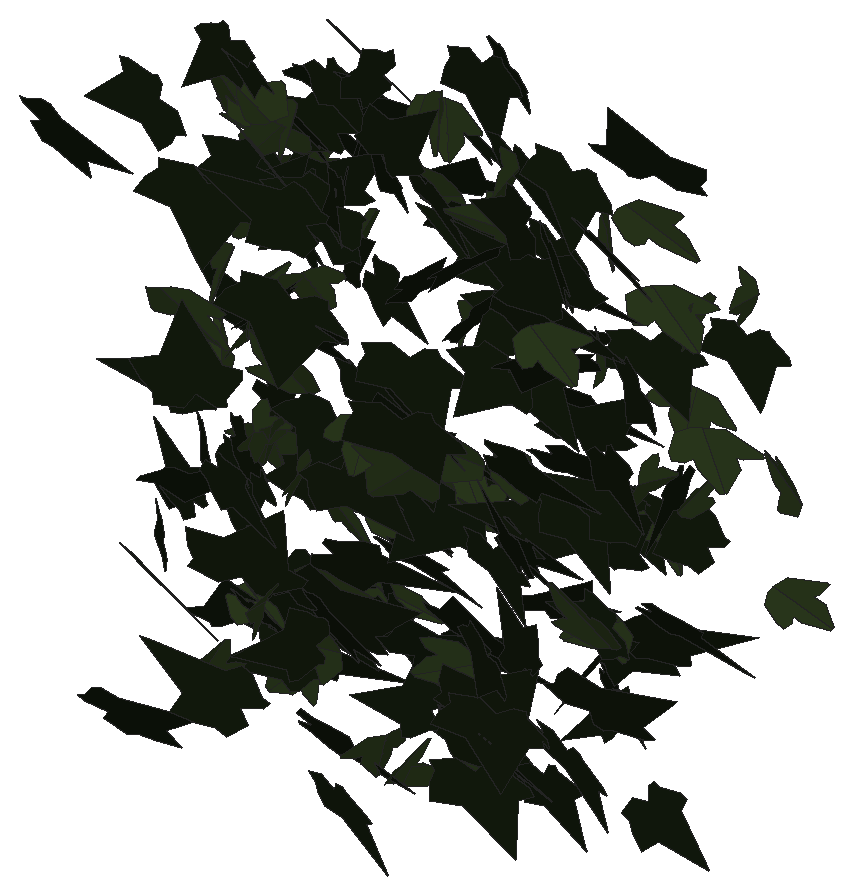
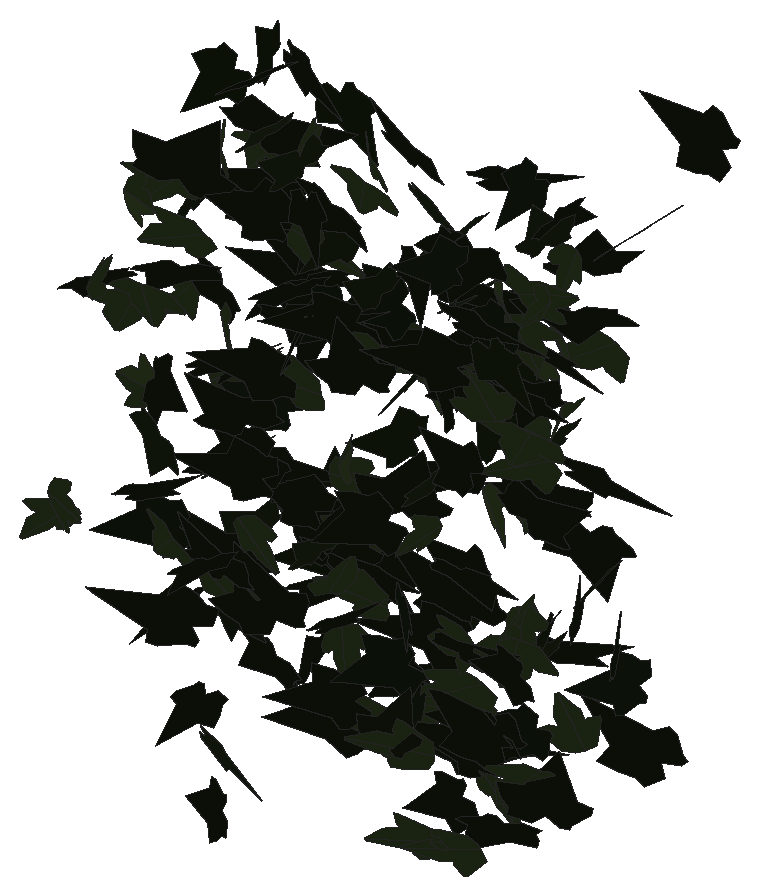
# SketchUp Ruby script. Lengths in millimetres.
U = 1.mm
M = Sketchup.active_model
def pt(a) = Geom::Point3d.new(a.map { |v| v * U })
def face(e, loops, mat)
  f = e.add_face(loops[0].map { |a| pt(a) })
  loops[1..].each { |l| e.add_face(l.map { |a| pt(a) }).erase! }
  f.material = f.back_material = mat if mat
  f
end
# faces: each face lists its corners as indices into pts; further lists are holes
def faces(e, pts, list, mat = nil) = list.each { |f| face(e, (f[0].is_a?(Array) ? f : [f]).map { |l| l.map { |i| pts[i] } }, mat) }
# xy, xz, yz: faces in a plane at the given z, y or x. An outline is a flat list of corners, or four numbers for a rectangle; further outlines are holes
def ring(l) = l.size == 4 ? [[l[0], l[1]], [l[2], l[1]], [l[2], l[3]], [l[0], l[3]]] : l.each_slice(2).to_a
def flat(e, list, mat, &to3) = list.each { |f| face(e, (f[0].is_a?(Array) ? f : [f]).map { |l| ring(l).map { |u, v| to3.(u, v) } }, mat) }
def xy(e, z, list, mat = nil) = flat(e, list, mat) { |x, y| [x, y, z] }
def xz(e, y, list, mat = nil) = flat(e, list, mat) { |x, z| [x, y, z] }
def yz(e, x, list, mat = nil) = flat(e, list, mat) { |y, z| [x, y, z] }
def lines(e, pts, list) = list.each { |a, b| e.add_line(pt(pts[a]), pt(pts[b])) }
# prism: a flat outline (further loops are holes) pulled along v
def prism(e, loops, v, mat = nil)
  f = face(e, loops, mat); d = Geom::Vector3d.new(v.map { |x| x * U })
  f.pushpull(f.normal.samedirection?(d) ? d.length : -d.length)
end
def box(e, o, s, mat = nil) = prism(e, [[o, [o[0] + s[0], o[1], o[2]], [o[0] + s[0], o[1] + s[1], o[2]], [o[0], o[1] + s[1], o[2]]]], [0, 0, s[2]], mat)
def at(x, y, z, deg = 0) = Geom::Transformation.translation(pt([x, y, z])) * Geom::Transformation.rotation(ORIGIN, Z_AXIS, deg.degrees)
def axes(o, x, y, z) = Geom::Transformation.new([*x, 0, *y, 0, *z, 0, *pt(o).to_a, 1])
def part(name) = M.definitions.add(name)
# library, detail: a bought-in or finely detailed component or shape, given as its bounding box
def library(name, o, s) = part(name).tap { |d| box(d.entities, o, s) }
def detail(e, o, s) = box(e.add_group.entities, o, s)
def put(e, d, t, mat = nil) = e.add_instance(d, t).tap { |i| i.material = mat if mat }
def group(e, t, mat = nil) = e.add_group.tap { |g| g.transformation = t; g.material = mat if mat }.entities
root = M.entities
M.materials.add("efeu1").color = [18, 25, 13]
M.materials.add("efeu2").color = [43, 57, 29]
c1 = part("ivyleaf_9")
p = [[39.1,54.8,31.7],[34.5,51.8,30.2],[-5.3,25.2,17.3],[-17.9,28.3,20.9],[-21.6,21.7,17],[-20.2,4.3,5.3],
  [-22.9,-0.3,2.5],[-17.1,-4,-0.6],[-2,-2.1,-1.2],[-0.7,-15.4,-10.1],[16.6,-22.3,-16.7],[21.1,-15.1,-12.5],
  [32.7,-10.7,-11],[46.1,-1.8,-6.6],[30.8,11.2,3.8]]
faces(c1.entities,p,[[0,1,2,3,4,5,6,7,8,9,10,11,12,13,14]],"efeu1")
c2 = part("ivyleaf_10")
p = [[0,12.8,-0.8],[-1.5,51.3,-10.9],[-4.9,51,-11.6],[-13.6,26.5,-7.3],[-13.2,15.9,-4.6],[-21.1,19.3,-7.2],
  [-29.5,16.3,-8.3],[-29.2,8.3,-6.2],[-19.7,-9.8,0.5],[-7.6,-13,4],[1,-12.2,5.8],[-0.4,51.1,-11.1],
  [-1.5,51.1,-10.9],[1,-12.4,5.9],[16.9,-12.4,3.5],[35.1,9.1,-5.1],[35,12.9,-6.1],[20.5,16.4,-4.9],
  [15.8,15,-3.8],[15.3,27.6,-7.1],[12.8,31.3,-7.8]]
faces(c2.entities,p,[[0,1,2,3,4,5,6,7,8,9,10],[11,12,0,13,14,15,16,17,18,19,20]],"efeu2")
put(root,c1,axes([5355,619.4,1867.7],[-0.14381,0.13814,1.11559],[-0.4553,-1.09447,0.11932],[2.0904,-0.22888,0.10273]))
put(root,c1,axes([5360.8,766.3,1691.6],[1.70624,0.24409,0.77946],[-1.42606,-0.21489,0.92911],[0.61874,-1.16838,-0.00805]))
put(root,c1,axes([5329.5,599.9,1839.7],[1.79661,-0.87085,0.22516],[0.30156,-0.16029,-1.28429],[1.68513,0.95714,-0.01022]))
put(root,c1,axes([5332.9,867,1972.2],[0.18817,-0.09167,-1.07306],[2.04965,0.00299,0.09898],[-0.01032,-1.0776,0.09155]))
put(root,c1,axes([5360,701.5,1966.5],[-0.00869,-0.12447,1.15708],[-0.36189,-1.14146,-0.12354],[2.1851,-0.18954,-0.01586]))
put(root,c1,axes([5352.7,875.9,1723.1],[-0.57705,-0.64679,-0.80667],[0.74353,0.70665,-0.71344],[1.82193,-0.49324,0.03566]))
put(root,c1,axes([5378.1,577.2,2538.2],[0.57772,-1.14595,-0.77761],[0.39902,-0.74886,1.18544],[-2.60531,-0.36881,0.00913]))
put(root,c1,axes([5408.1,745.4,2149.6],[0.33354,-0.23641,1.17944],[-1.48326,0.88558,0.29331],[-1.74387,-0.79845,-0.0239]))
put(root,c2,axes([5356,812.5,2329.7],[2.19955,0.23269,0.39445],[0.73662,0.0761,-1.1789],[-0.46594,1.2188,-0.0017]))
put(root,c1,axes([5381.4,737.3,1975.6],[1.09422,-0.48773,-0.98454],[-1.42174,0.64132,-0.75394],[1.53341,0.94265,0.00353]))
put(root,c2,axes([5362.2,782.7,2273.4],[-0.9382,-0.24559,-0.99546],[1.69083,0.44907,-0.55074],[0.97411,-1.01601,-0.0028]))
put(root,c2,axes([5397.6,665.5,2546.6],[-1.50843,0.82441,0.15893],[-0.20941,0.11468,-1.1436],[-1.58412,-0.80018,-0.00016]))
put(root,c2,axes([5397.7,792.7,1959.3],[-2.09417,-0.35277,-0.11717],[0.2135,0.03391,-1.15551],[0.67448,-1.10604,0.00195]))
put(root,c1,axes([5445.6,583.6,2140.5],[-1.49062,0.32897,0.81601],[-1.45656,0.28421,-0.84914],[-0.82606,-1.09477,0.02476]))
put(root,c1,axes([5361.6,946.1,2331.5],[1.3684,-0.14985,-0.80959],[1.52545,-0.11846,0.73375],[-0.35842,-1.07627,0.03197]))
put(root,c1,axes([5417.4,599.1,1962.1],[-0.60237,-0.95514,0.7801],[0.42008,0.7485,1.00601],[-2.30919,0.38532,-0.02049]))
put(root,c1,axes([5386.5,752.3,1928.9],[-0.03808,-0.98467,0.67121],[-0.046,-0.67083,-0.98484],[2.26754,-0.03015,-0.00871]))
put(root,c1,axes([5433.7,702,2403.7],[-2.0111,0.13155,0.15533],[-0.29362,0.01806,-1.06485],[-0.25271,-1.0679,0.00113]))
put(root,c2,axes([5403.7,706.1,2492.9],[-0.13421,0.41004,1.10293],[-0.29642,1.09193,-0.41591],[-2.21976,-0.1706,-0.01115]))
put(root,c1,axes([5359.7,512.3,1667.6],[2.21567,0.25602,-0.50333],[0.86821,0.2534,1.18402],[0.63347,-1.24276,0.13773]))
put(root,c2,axes([5440.2,708.3,2490],[1.51976,0.04929,0.98333],[-1.87076,-0.03251,0.79985],[0.10719,-1.26631,0.01774]))
put(root,c2,axes([5415.3,756.2,1987.9],[-0.37265,-1.16254,-0.2124],[0.13303,0.20353,-1.17841],[2.24523,-0.20501,0.03457]))
put(root,c1,axes([5431,803.6,2441.7],[-0.64392,1.01158,-0.43434],[0.18536,-0.42511,-1.06593],[-2.08699,-0.34987,0.03934]))
put(root,c2,axes([5393.3,759.4,1739.4],[1.19414,0.88081,0.55524],[0.59722,0.45816,-1.08139],[-1.88949,0.70147,0.00911]))
put(root,c2,axes([5383.7,925.3,1694.2],[-0.69017,-0.14399,-1.02714],[1.90192,0.24278,-0.38685],[0.52843,-1.06188,0.05083]))
put(root,c2,axes([5412.4,741.2,1996.5],[0.1379,-0.47808,-1.15184],[0.59001,1.12448,-0.44722],[2.29902,-0.25991,0.18386]))
put(root,c2,axes([5447.8,732.9,2448.4],[-1.82548,-0.49863,0.44577],[-0.75952,-0.19875,-1.081],[1.0215,-1.03885,-0.00715]))
put(root,c1,axes([5424.9,774.4,2365],[-1.9216,-0.48929,-0.54058],[0.92024,0.2418,-1.12196],[1.03867,-1.11946,-0.00607]))
put(root,c1,axes([5426.7,662.3,2599.2],[0.30826,-0.2751,-1.16488],[0.86532,-1.07324,0.31668],[-2.10723,-0.48096,-0.04037]))
put(root,c1,axes([5374.8,354,2600.6],[1.68405,-0.15593,-1.12311],[2.15668,0.07154,0.88285],[-0.07584,-1.42802,0.16687]))
put(root,c1,axes([5416.2,736,2330.6],[-0.82843,-0.2475,1.05029],[1.92139,0.30648,0.49062],[-0.72514,1.09483,0.10009]))
put(root,c2,axes([5427.4,815.2,2353.3],[-1.04265,-0.94769,0.22801],[0.28668,0.1761,1.09386],[-1.83282,0.56666,0.04139]))
put(root,c1,axes([5428.6,674.2,1938.7],[0.92724,-0.58893,-0.7975],[-0.88294,0.64986,-0.76332],[1.66747,0.6716,0.03928]))
put(root,c1,axes([5449.9,554.9,2024.9],[0.83795,0.9579,-0.52718],[-0.39817,-0.48401,-1.05419],[-2.04248,0.48734,-0.01078]))
put(root,c1,axes([5436.5,606.6,2418.2],[-1.40768,-1.12135,-0.34748],[0.34435,0.2969,-1.34326],[2.20757,-0.76135,-0.01205]))
put(root,c1,axes([5425.8,685.9,2572],[-0.21824,-0.79523,0.86357],[0.44009,-0.86598,-0.76674],[2.19047,0.09475,0.24009]))
put(root,c2,axes([5440.9,595.2,1712.1],[-0.6345,-1.21557,0.09661],[0.13109,0.08123,1.25966],[-2.31707,0.33747,0.04481]))
put(root,c1,axes([5493,794.4,1921.1],[-2.2889,-0.16025,-0.31583],[-0.58957,-0.06593,1.21306],[-0.3267,1.24169,0.02365]))
put(root,c1,axes([5434.4,788.9,2278.7],[0.17725,-0.79028,0.87266],[0.31566,-0.85785,-0.79456],[2.21832,0.18521,0.04333]))
put(root,c1,axes([5441.8,694,1769.9],[1.94462,-0.26445,-0.33045],[-0.60717,0.08621,-1.05543],[0.52933,1.0704,0.00336]))
put(root,c1,axes([5448.7,756.9,2463.2],[1.84421,-0.27585,-0.4644],[-0.86096,0.10675,-1.00732],[0.56175,1.06923,-0.01925]))
put(root,c1,axes([5507.6,773.7,2451],[-1.04749,0.39051,0.93386],[-1.58409,0.43033,-0.6705],[-1.09632,-0.9949,0.07654]))
put(root,c2,axes([5458.8,666.4,2235.3],[0.07369,-0.83175,0.95346],[-0.07083,0.95274,0.83264],[-2.40701,-0.0535,0.00469]))
put(root,c2,axes([5482.8,735,1681.5],[1.78951,-0.67287,-0.48666],[-0.68996,0.32881,-1.15506],[1.4219,1.00639,0.052]))
put(root,c2,axes([5471.6,731.7,2481.9],[1.05989,-0.95333,0.35906],[0.44469,-0.27876,-1.10254],[1.88711,0.60112,0.05814]))
put(root,c2,axes([5442.9,938,1692.9],[0.67606,0.24862,1.05811],[1.72269,0.54863,-0.43278],[-1.14526,0.972,-0.02637]))
put(root,c1,axes([5475.6,821.5,1701.4],[-0.07252,0.70891,-0.91126],[-0.51028,0.8814,0.69689],[2.13724,0.23449,0.13547]))
put(root,c1,axes([5511.2,700.8,1713.9],[-1.2349,-0.30352,0.79751],[-1.27735,-0.43718,-0.71245],[1.00291,-0.93054,0.07458]))
put(root,c2,axes([5494.2,558.6,2203.4],[0.13729,0.95274,-0.69451],[-0.03301,0.69659,0.95379],[2.24363,-0.04805,0.05653]))
put(root,c2,axes([5466.1,506.6,2308.4],[-1.85622,0.22209,-0.70933],[1.32527,-0.13632,-1.00013],[-0.49482,-1.19825,-0.01769]))
put(root,c1,axes([5490.8,820.8,2336],[0.1382,-0.33673,1.16286],[0.84276,1.09162,0.28845],[-2.14442,0.40731,0.18831]))
put(root,c2,axes([5488.9,578.6,2345.8],[0.98997,-1.0802,0.39426],[0.36451,-0.34529,-1.19872],[2.15793,0.55388,0.02161]))
put(root,c1,axes([5456,860.7,2434.5],[1.17333,0.11599,0.96774],[1.8077,0.18537,-0.62731],[-0.4161,1.13235,0.00356]))
put(root,c1,axes([5460.1,754.7,1764.8],[1.81309,0.74399,-0.18717],[0.28053,0.11536,1.20875],[1.43288,-0.96399,0.00019]))
put(root,c1,axes([5476.6,787.5,2348.9],[-0.64554,-0.14159,1.12986],[2.12229,0.19735,0.35949],[-0.43871,1.16305,0.07655]))
put(root,c1,axes([5514.4,767.3,2035.4],[-1.9924,-0.2994,-0.37019],[0.67515,0.10588,-1.08883],[0.60436,-1.10533,-0.00403]))
put(root,c2,axes([5481.7,914.9,1816.5],[0.03747,-0.0615,1.20762],[1.75604,0.78139,0.02475],[-1.48741,0.92096,0.05964]))
put(root,c1,axes([5519.2,740.1,2550.3],[1.70878,0.56934,-0.29116],[-0.46698,-0.15675,-1.06314],[-1.12389,0.93077,-0.00095]))
put(root,c1,axes([5482.1,740,1776.2],[0.10803,-0.27807,-1.22493],[2.30531,0.33674,-0.02031],[0.6329,-1.17911,0.28308]))
put(root,c1,axes([5491.9,816.9,2564.2],[1.51219,-0.80897,0.29888],[0.39092,-0.21719,-1.1339],[1.59413,0.82066,-0.00546]))
put(root,c1,axes([5528.1,921.6,1816.6],[1.53646,-0.80675,0.17196],[-0.22187,0.1266,1.14129],[-1.55415,-0.81565,0.00707]))
put(root,c1,axes([5528.3,589.7,2274.9],[0.75615,0.84233,1.09244],[0.81592,1.00515,-0.93094],[-2.4954,0.5839,0.02664]))
put(root,c1,axes([5576.3,490.7,1763.1],[-1.85382,-0.75088,-0.3496],[-0.5109,-0.22436,1.22981],[-1.49129,1.01028,0.01327]))
put(root,c2,axes([5568.6,681.9,1758.1],[0.85316,-0.4072,-1.07917],[-1.4702,0.75381,-0.60532],[1.6302,0.89293,0.01887]))
put(root,c2,axes([5513.4,769.2,1919.7],[-0.93961,0.47605,-0.95253],[1.2306,-0.70018,-0.68507],[-1.61024,-0.81289,0.03226]))
put(root,c2,axes([5546.5,544.3,2276.4],[0.00193,-0.88238,-0.79292],[-0.05388,0.79268,-0.88215],[2.25713,0.01968,-0.02038]))
put(root,c1,axes([5498.2,715.5,1716.5],[1.22832,-0.18853,1.0595],[1.95342,-0.26347,-0.67211],[0.61557,1.21229,0.0187]))
put(root,c2,axes([5524.4,741.7,1829.5],[-1.36424,-0.28568,-1.00092],[1.81803,0.3022,-0.77036],[0.78691,-1.19346,0.04452]))
put(root,c2,axes([5554.1,663.4,2301.8],[-1.31998,-0.7258,-0.49517],[0.63998,0.36355,-1.00387],[1.54488,-0.77074,-0.00722]))
put(root,c1,axes([5541.9,723,2568],[0.85221,-1.08533,-0.28321],[-0.2342,0.25557,-1.17396],[2.12187,0.46411,-0.01583]))
put(root,c2,axes([5561.1,782.4,2336.2],[0.80216,-0.93148,0.54692],[0.39921,-0.50532,-1.02229],[2.01665,0.47054,-0.01518]))
put(root,c2,axes([5562.1,781.4,2092.5],[-0.04276,0.4161,1.06815],[-0.11629,1.0664,-0.41671],[-2.17861,-0.06509,0.00128]))
put(root,c1,axes([5574.6,791.2,1815.2],[1.12683,-0.39384,-0.90621],[-1.45271,0.48855,-0.71103],[1.19417,0.96596,-0.00987]))
put(root,c1,axes([5595.8,659.9,2420.3],[-1.93584,-0.6559,0.31728],[-0.50955,-0.17025,-1.21029],[1.28968,-1.0518,-0.00195]))
put(root,c1,axes([5556.6,741,2296.2],[-0.04211,0.48515,1.08373],[0.12267,-1.08183,0.48561],[2.25646,0.06787,-0.00618]))
put(root,c1,axes([5569.4,534.8,2556.5],[1.80409,-0.38331,-0.6102],[-1.04332,0.27085,-1.02174],[0.89015,1.09433,0.03915]))
put(root,c2,axes([5613,563.4,2216.8],[-1.7619,0.25651,-0.71186],[-1.29894,0.2026,0.96058],[0.62179,1.1501,-0.01044]))
put(root,c2,axes([5587.3,611.2,2058.4],[0.52257,-1.22543,-0.08057],[-0.03337,0.07864,-1.25581],[2.33703,0.27513,0.00009]))
put(root,c1,axes([5567.1,471.6,2107.2],[1.16642,-0.98298,-0.43993],[-0.41623,0.38203,-1.15829],[2.00692,0.65054,0.01546]))
put(root,c1,axes([5616.2,778.4,1958.2],[-0.26618,0.12386,-1.10353],[-1.70436,0.64509,0.1859],[1.24967,0.90619,0.01849]))
put(root,c1,axes([5626.6,721.9,2594.5],[-1.60188,0.82454,-0.07064],[0.0965,-0.04918,-1.17825],[-1.57205,-0.8432,-0.00035]))
put(root,c1,axes([5597.2,679.6,2409.9],[-0.07537,-0.2197,1.25326],[-0.68453,-1.20079,-0.22187],[2.32281,-0.361,-0.02472]))
put(root,c1,axes([5614.7,658.7,2390.9],[0.259,-1.07513,-0.30959],[0.07902,-0.3068,1.08371],[-2.12787,-0.14225,0.00256]))
put(root,c1,axes([5570.8,708.9,1882.4],[0.77481,0.39237,-1.14031],[1.38945,0.87774,0.56266],[1.82675,-0.83404,0.05569]))
put(root,c1,axes([5629.7,340.3,2306.8],[-1.8109,-0.69548,0.84528],[1.30818,0.49202,1.17856],[-1.62132,1.17379,0.00681]))
put(root,c1,axes([5655.7,546.5,1853],[-1.86562,0.91032,0.12526],[-0.17653,0.08419,-1.33775],[-1.7399,-0.98463,0.00142]))
put(root,c1,axes([5593.6,731.8,2137],[0.7158,-1.26099,0.13977],[0.06769,-0.13524,-1.31587],[2.41366,0.37776,-0.00455]))
put(root,c1,axes([5612.4,459,1980.5],[-1.76181,0.02936,0.96233],[1.81541,-0.15319,0.92224],[0.24865,1.32648,0.08521]))
put(root,c1,axes([5641.5,710.6,2476.9],[1.10402,-0.15207,-1.03385],[-1.90046,0.26783,-0.59968],[0.58614,1.15482,0.00294]))
put(root,c1,axes([5611.2,878.9,2364.5],[1.91274,0.36415,0.33832],[-0.60698,-0.11293,1.06895],[0.7256,-1.0544,0.00236]))
put(root,c1,axes([5597.7,795.4,1865.1],[2.13972,-0.23516,0.17058],[0.31587,-0.03968,-1.1486],[0.45379,1.13645,-0.00481]))
put(root,c1,axes([5588,640.6,1667.2],[1.84497,-0.51651,0.58443],[0.97251,-0.28379,-1.09838],[1.1215,1.0958,-0.00898]))
put(root,c1,axes([5630.2,534.7,2348.1],[-1.61151,-1.13287,-0.29785],[0.39133,0.21806,-1.41395],[2.19473,-0.87071,0.03341]))
put(root,c2,axes([5655.7,827.6,2385.6],[1.27185,-0.3653,-0.84733],[-1.02544,0.69484,-0.7245],[1.42563,0.82569,0.23481]))
put(root,c1,axes([5603.6,566.7,2292.9],[2.10027,-0.07825,-0.48047],[0.91367,-0.02228,1.10626],[-0.15348,-1.2034,0.01076]))
put(root,c1,axes([5682.3,490.1,2501.4],[-1.43237,-0.8667,-0.49716],[-0.62335,-0.37403,1.14787],[-1.79655,0.82079,-0.0019]))
put(root,c1,axes([5629.9,712.9,2305.8],[1.18466,-0.80782,-0.77802],[-0.88194,0.62507,-1.01975],[1.94383,0.77592,0.01149]))
put(root,c1,axes([5653.4,728.3,2074.3],[1.76536,0.02353,0.73982],[-1.40832,0.00048,0.92775],[0.03443,-1.18648,0.01505]))
put(root,c2,axes([5648.6,459.8,1948.3],[-0.23771,-0.39467,-1.17949],[-0.15162,-1.18045,0.40343],[-2.36228,0.11548,0.0928]))
put(root,c1,axes([5684.3,870.2,1931],[-0.81278,-1.03566,-0.02438],[0.09221,-0.04631,1.11851],[-1.96946,0.42524,0.06243]))
put(root,c1,axes([5639.7,723.5,1824.2],[-0.34776,-0.08494,-1.09194],[2.07179,-0.13599,-0.17158],[-0.22953,-1.09874,0.10565]))
put(root,c1,axes([5628.9,611.7,1861],[-0.22793,0.04414,1.44843],[2.12848,-0.92139,0.12055],[1.75378,1.12398,0.04194]))
put(root,c2,axes([5664.8,850.1,2198],[0.05019,-0.19723,1.09826],[1.0024,-0.96628,-0.18617],[1.87218,0.52265,0.07024]))
put(root,c1,axes([5659.7,606.2,2080.6],[-0.02042,-0.71778,-1.04212],[0.39524,1.02703,-0.70952],[2.37565,-0.17704,0.10909]))
put(root,c1,axes([5657.2,767.9,2069.5],[2.21018,-0.09629,0.1445],[0.2712,-0.02989,-1.16514],[0.18884,1.16987,-0.01788]))
put(root,c1,axes([5710.7,763.9,1974.1],[-2.45608,-0.23851,-0.15091],[0.28481,0.02066,-1.31234],[0.45545,-1.29913,0.00684]))
put(root,c2,axes([5649.7,801.8,1953.9],[0.09202,-0.0712,1.16573],[2.21168,0.11926,-0.04091],[-0.22161,1.16062,0.07572]))
put(root,c1,axes([5649.2,572.8,1886.7],[1.35304,-0.19479,-1.06053],[1.98017,-0.2096,0.73596],[-0.5388,-1.25945,0.04154]))
put(root,c2,axes([5701.6,631.7,1693],[-0.71774,-1.18981,-0.14183],[0.08995,0.13381,-1.24813],[2.2787,-0.38004,0.00459]))
put(root,c1,axes([5673.8,758.7,2433.6],[0.70416,-1.0058,0.46898],[0.26703,-0.44799,-1.07148],[2.09515,0.39514,-0.02106]))
put(root,c2,axes([5709.5,812.1,1961.1],[0.91006,1.09039,0.05461],[-0.06878,-0.04378,1.19053],[2.0767,-0.47929,0.0155]))
put(root,c1,axes([5669.5,693.4,2166.1],[1.54344,-0.98195,0.20389],[0.24677,-0.15736,-1.27354],[1.8927,0.82127,-0.00023]))
put(root,c2,axes([5707.8,659.2,1633],[0.13494,-1.03758,0.44217],[0.06474,0.44481,1.03831],[-2.14558,-0.05183,0.05914]))
put(root,c1,axes([5738.6,677.5,1731.5],[-0.4464,-0.15229,1.13008],[-1.70371,-0.69008,-0.27879],[1.34432,-0.92514,0.02194]))
put(root,c2,axes([5761.9,721.2,2084.2],[-0.13095,0.08761,-1.19349],[-2.24369,0.20046,0.08268],[0.39137,1.17855,0.07465]))
put(root,c1,axes([5739.4,841.9,2596.1],[0.90021,-0.04615,-1.08266],[-2.00128,0.26586,-0.47074],[0.49828,1.15117,0.06531]))
put(root,c1,axes([5706.3,785.5,2526.8],[1.75503,-0.49704,-0.47016],[-0.64572,0.35299,-1.03862],[1.13073,0.97304,0.13662]))
put(root,c1,axes([5711,822.3,2593.6],[-1.43026,-0.08358,-1.09621],[2.09088,-0.00723,-0.7526],[0.07857,-1.32905,0.07303]))
put(root,c1,axes([5701.8,786.6,2389.2],[0.31592,0.36104,-1.12492],[1.03319,0.98563,0.39645],[1.99707,-0.56703,-0.02715]))
put(root,c2,axes([5724,726.7,2577],[2.07467,-0.27328,0.37392],[0.6739,-0.12459,-1.12334],[0.56816,1.14569,-0.03297]))
put(root,c1,axes([5725.4,651.2,2352.1],[0.87392,0.52009,1.16295],[1.34612,0.92408,-0.69253],[-2.01656,0.84224,0.0417]))
put(root,c1,axes([5703.5,785.3,1765.3],[1.77692,-0.02453,0.62165],[1.17982,-0.05792,-0.93333],[0.09992,1.12018,-0.03464]))
put(root,c1,axes([5726,609.2,2567.8],[-0.86394,0.82052,0.827],[0.78242,-0.71764,0.93767],[2.07455,0.61236,-0.00924]))
put(root,c2,axes([5744.8,545.5,2199.7],[1.6834,0.78328,-0.26797],[-0.37769,-0.1801,-1.18147],[-1.52962,0.9065,-0.00318]))
put(root,c1,axes([5779.7,780.7,2351.8],[-1.29369,-0.94569,-0.23585],[-0.23396,-0.20206,1.1645],[-1.84015,0.69054,0.01776]))
put(root,c2,axes([5735,697.3,2604.1],[1.10919,-0.71904,0.76407],[1.00158,-0.5558,-0.92445],[1.72748,0.78393,0.04539]))
put(root,c1,axes([5745.2,635.2,2259.8],[-0.7673,-1.07731,-0.59291],[0.53218,0.5273,-1.14824],[2.27904,-0.48584,0.06851]))
put(root,c2,axes([5778.4,709,1813.2],[-0.77958,-1.06961,-0.20252],[0.14597,0.18749,-1.14535],[2.0667,-0.41671,0.0045]))
put(root,c2,axes([5779.8,655.2,1666],[-1.6289,-0.53018,-0.63583],[0.99943,0.35932,-1.00648],[1.21805,-1.00383,-0.02446]))
put(root,c1,axes([5762.9,462.9,1711.7],[0.90579,-1.16558,0.30315],[0.21912,-0.28043,-1.259],[2.28163,0.48966,0.00056]))
put(root,c2,axes([5841.7,720.1,2447.4],[-0.47604,0.05133,1.18971],[-2.26124,-0.09251,-0.2458],[0.15241,-1.2122,0.06914]))
put(root,c1,axes([5808.7,676.6,2328],[-0.45008,0.46146,-1.19729],[-0.97209,1.08299,0.51829],[2.24025,0.56264,-0.01565]))
put(root,c1,axes([5807.2,759.2,2354.6],[0.85419,-0.44443,-1.11754],[-1.52815,0.77732,-0.6316],[1.7041,0.91984,-0.00622]))
put(root,c1,axes([5765.9,736.4,1683.7],[0.05018,-0.25974,-1.18812],[1.9851,0.61599,-0.11152],[1.19035,-1.01631,0.23606]))
put(root,c1,axes([5777.4,994.4,1650.5],[0.27233,-0.02543,-1.18926],[2.16239,-0.35177,0.14423],[-0.67038,-1.14502,-0.0179]))
put(root,c1,axes([5776.8,612.1,1853.2],[0.04318,-0.11814,1.26139],[2.40638,0.08161,-0.0151],[-0.15193,1.25895,0.11935]))
put(root,c2,axes([5845.9,498,2193.4],[-1.97225,-0.16877,0.63948],[-1.1801,-0.1656,-1.04852],[0.4379,-1.20639,0.05447]))
put(root,c1,axes([5799.1,736.1,1955.2],[0.37878,-1.14757,0.3867],[0.20436,-0.37362,-1.16402],[2.29565,0.22261,0.03982]))
put(root,c1,axes([5806.2,541.7,2231.4],[-1.48846,-0.5897,-0.96526],[1.48622,0.56749,-0.97942],[1.55743,-1.10514,0.01213]))
put(root,c1,axes([5865.8,726.9,2324.8],[-1.92608,-0.59753,0.14505],[-0.23842,-0.07311,-1.17526],[1.1457,-1.01975,-0.00073]))
put(root,c1,axes([5845.3,640.2,1888.9],[1.99521,-0.6352,0.39659],[-0.63863,0.21149,1.22575],[-1.27409,-1.10072,0.00666]))
put(root,c2,axes([5873,809,1997.6],[1.08084,-0.30836,-0.97559],[-1.13873,0.80503,-0.60275],[1.57962,0.79133,0.23302]))
put(root,c1,axes([5878,891.6,1683.8],[-1.55845,0.74891,-0.2525],[0.33535,-0.18144,-1.10959],[-1.4663,-0.83747,0.0146]))
put(root,c1,axes([5812.9,862.1,2127.9],[1.46211,-0.32958,0.76916],[1.37098,-0.27086,-0.83555],[0.81041,1.05282,0.02582]))
put(root,c2,axes([5885.9,572.3,1895.2],[1.64459,-0.34512,-0.80747],[-1.4578,0.25775,-0.92987],[0.81726,1.15424,-0.03379]))
put(root,c1,axes([5838.1,796.3,1860.8],[2.10818,0.60197,0.32902],[-0.54982,-0.15746,1.2607],[1.18421,-1.14476,-0.00039]))
put(root,c1,axes([5838,788.8,2261.6],[0.66783,0.70583,-0.82974],[0.5784,0.77369,0.78667],[1.99093,-0.46153,0.04978]))
put(root,c1,axes([5833.4,712.2,2002.5],[0.85812,-0.42977,0.99442],[1.29063,-0.72801,-0.62211],[1.60785,0.81375,-0.03136]))
put(root,c1,axes([5871.5,916.2,1769.4],[0.15334,-0.26114,-1.21709],[-0.78781,1.14461,-0.27299],[2.23426,0.42151,-0.01273]))
put(root,c1,axes([5850.5,714.4,2561.3],[0.90778,-1.23547,0.3499],[0.21297,-0.33185,-1.32426],[2.43453,0.48971,-0.01462]))
put(root,c1,axes([5933.6,718.3,2044.5],[-1.33079,-0.0748,1.06041],[-2.01069,-0.092,-0.70313],[0.22458,-1.26686,-0.01155]))
put(root,c2,axes([5878.4,670.3,2564.5],[-0.06305,0.02076,1.20918],[0.89222,-1.11483,0.03198],[2.12168,0.46943,0.02248]))
put(root,c1,axes([5876.8,901.5,1984.1],[0.19064,-1.00887,-0.62351],[-0.13397,0.61957,-1.0138],[2.25321,0.1222,-0.00752]))
put(root,c1,axes([5904.6,624.6,1683.7],[-0.51579,-0.59138,1.26391],[1.08399,1.12851,0.65016],[-2.42446,0.63038,0.0218]))
put(root,c1,axes([5909.8,969.6,2206.8],[0.2396,0.78452,0.91321],[0.18093,0.90885,-0.79387],[-2.28415,0.15428,0.03291]))
put(root,c1,axes([5914.3,615.7,2310.5],[-1.25043,-0.8236,0.4983],[-0.52187,-0.41818,-1.05272],[1.75613,-0.7107,0.04197]))
put(root,c1,axes([5885.4,853.9,1943.1],[-0.88558,0.47847,0.92349],[1.13709,-0.70516,0.66638],[1.6203,0.75637,0.03708]))
put(root,c1,axes([5873.2,774.1,2104.8],[2.15683,0.12166,0.35642],[0.68002,0.00994,-1.13946],[-0.22658,1.18795,-0.02697]))
put(root,c2,axes([5940,790.6,1877.5],[1.72624,-0.41078,-0.67371],[-1.176,0.26861,-0.99567],[0.93396,1.09746,-0.00848]))
put(root,c1,axes([5908.8,776,2147.6],[-0.71484,-0.17962,1.12155],[2.13167,0.13775,0.39716],[-0.35927,1.17472,0.12492]))
put(root,c1,axes([5954.2,493.6,2543],[-0.3102,1.13065,-0.45165],[0.13657,-0.44597,-1.14231],[-2.31315,-0.17795,-0.00687]))
put(root,c1,axes([5943.9,768,1838.9],[-0.93457,0.574,-0.91898],[1.02737,-0.74522,-0.75392],[-1.788,-0.72822,0.04715]))
put(root,c2,axes([5893.5,647.2,2149.1],[0.39175,-0.10939,1.19448],[2.2819,0.05365,-0.2017],[-0.06571,1.2109,0.11685]))
put(root,c1,axes([5895.8,540.5,1828.8],[2.11298,-0.72334,0.32374],[0.52149,-0.17249,-1.32507],[1.41524,1.14353,0.00491]))
put(root,c1,axes([5922.7,643.2,2306.9],[0.27652,-1.13487,-0.69457],[-0.01016,0.6982,-1.14191],[2.53228,0.12673,0.07126]))
put(root,c2,axes([5961.4,752.2,2284.7],[0.11632,-0.26829,-1.15406],[-0.50057,1.12369,-0.27516],[2.19872,0.27002,-0.00159]))
put(root,c1,axes([5974.4,575.5,1926.7],[0.01615,0.13135,1.30354],[-0.36604,1.28957,-0.12869],[-2.46644,-0.19052,0.02763]))
put(root,c1,axes([5937.7,547.6,1935.4],[-0.13263,-0.72711,1.04143],[-0.23532,-1.03416,-0.73031],[2.40586,-0.14124,-0.01402]))
put(root,c1,axes([5934.9,532.6,1768.5],[-0.39081,-1.15684,-0.58674],[0.35274,0.56179,-1.1725],[2.44337,-0.26613,0.07542]))
put(root,c1,axes([5939.2,538.9,1854.9],[-1.38592,0.39761,0.96343],[1.61327,-0.45791,0.82968],[1.15417,1.1175,-0.00282]))
put(root,c1,axes([5936.8,669.5,1704.9],[-0.68438,-0.07566,-1.07282],[2.03173,0.11214,-0.36573],[0.24836,-1.12591,0.03566]))
put(root,c1,axes([6012.4,529.3,2600.4],[-0.39429,0.08595,-1.22035],[-2.29407,0.19721,0.21852],[0.39794,1.222,0.05057]))
put(root,c2,axes([5946.4,892.9,1989.3],[1.61748,-0.42418,0.82528],[1.39198,-0.38249,-0.94978],[1.08681,1.12119,-0.01179]))
put(root,c1,axes([5927.2,677.8,2429.4],[1.18727,-0.5405,0.88863],[1.4927,-0.43611,-0.81586],[1.30012,0.9943,0.12522]))
put(root,c1,axes([5992.9,818,2541.3],[1.79848,-0.33268,0.91408],[-1.60148,0.35977,1.00085],[-0.92878,-1.26455,0.04426]))
put(root,c1,axes([5977.3,516.2,1875.5],[-1.39555,-0.83517,-0.53296],[0.67696,0.39692,-1.11138],[1.75985,-0.81497,0.00488]))
put(root,c1,axes([6038.2,566.5,2483.4],[0.02882,0.07865,1.42004],[-2.42858,0.62783,-0.02117],[-1.19522,-1.2738,0.07725]))
put(root,c1,axes([6016.8,513,2118.9],[0.15849,-0.59828,1.07913],[-0.37959,1.06084,0.60353],[-2.31744,-0.21468,-0.02505]))
put(root,c1,axes([5943.1,607.3,2431.6],[0.78845,-0.11876,-1.276],[2.26099,0.53849,0.33558],[0.91465,-1.22875,0.2704]))
put(root,c1,axes([5954.1,848.5,1829.8],[0.61944,-0.00545,1.28688],[2.41789,0.21297,-0.32041],[-0.39045,1.31021,0.05744]))
put(root,c2,axes([5962.1,828.8,2460.3],[1.2142,0.15904,0.93735],[1.61261,0.41693,-0.64743],[-0.82077,1.05443,0.11462]))
put(root,c1,axes([6016.8,573.9,2383.3],[0.65087,1.13401,-0.50168],[-0.31881,-0.47339,-1.18426],[-2.33839,0.38019,0.02182]))
put(root,c1,axes([5991.3,622.6,2522.7],[0.10692,-1.10787,0.34564],[0.01772,-0.34561,-1.10927],[2.20867,0.0564,-0.00783]))
put(root,c1,axes([6002.5,639.5,2620],[-0.42672,-1.31463,0.26561],[-0.11359,-0.25925,-1.33353],[2.55003,-0.23154,-0.01496]))
put(root,c1,axes([6053.4,844.7,2009.3],[-1.23085,-0.95272,-0.09064],[-0.05921,-0.08841,1.15124],[-1.82044,0.64704,0.02384]))
put(root,c1,axes([5985.1,586.7,2056.7],[1.08874,-0.87365,0.76184],[0.97986,-0.56967,-1.03987],[1.97658,0.76363,0.09586]))
put(root,c1,axes([5979.7,529.7,2244],[1.10994,0.12374,-1.09187],[2.00597,0.2866,0.59545],[0.59146,-1.20423,0.02952]))
put(root,c2,axes([6006.2,701.8,2527.3],[0.51291,-0.59009,1.02367],[1.41074,-0.73322,-0.61781],[1.75122,0.76349,0.19787]))
put(root,c1,axes([6014.5,629.2,2143],[0.23025,-1.28378,-0.24874],[-0.04421,0.24765,-1.28947],[2.48834,0.12319,0.00011]))
put(root,c1,axes([6048.5,659.7,1968],[0.25053,-1.06979,-0.31163],[0.07755,-0.30896,1.07786],[-2.11924,-0.13777,0.0026]))
put(root,c1,axes([6068.7,669.7,2136.6],[-0.72255,-1.06536,-0.4059],[-0.0927,-0.41227,1.12762],[-2.16779,0.37272,0.08707]))
put(root,c1,axes([6012.5,671.7,1830.1],[-0.39205,-0.17401,1.28979],[2.17733,-0.6468,0.09546],[1.18094,1.13475,0.25219]))
put(root,c1,axes([6047.7,747.6,2340.5],[-0.56212,-0.97904,-0.61849],[0.56381,0.55317,-1.01712],[2.13064,-0.40468,0.10598]))
put(root,c2,axes([6094.8,970.2,2042.9],[-0.14849,0.12604,-1.2232],[-1.12001,1.07236,0.14804],[2.0549,0.59359,-0.0077]))
put(root,c2,axes([6050.2,517.9,2450.2],[1.114,0.96556,0.5108],[0.46134,0.45025,-1.12887],[-2.02712,0.63309,0.0238]))
put(root,c1,axes([6037.3,773.8,1929.7],[2.08342,-0.34863,0.37768],[0.69906,-0.09101,-1.14863],[0.68429,1.15443,0.02351]))
put(root,c1,axes([6052.3,571.7,1824.7],[0.53787,-1.21211,0.68621],[0.33146,-0.66395,-1.24452],[2.63012,0.33156,0.01651]))
put(root,c1,axes([6082.3,761.1,2149.2],[-0.65554,0.40732,-1.32647],[1.62527,-1.01502,-0.53343],[-2.08153,-0.92081,0.00124]))
put(root,c2,axes([6119.7,545.4,2030.4],[-1.71355,0.47876,-0.7305],[-1.33431,0.22951,1.01452],[0.99131,1.13648,0.10285]))
put(root,c1,axes([6060.2,523.9,2586.3],[0.6717,-0.29697,-1.23892],[2.01409,-0.64746,0.45666],[-1.35004,-1.11368,0.06487]))
put(root,c2,axes([6091.1,890.2,2362.3],[-0.25327,0.26768,1.12161],[0.75369,-1.04978,0.29752],[2.06112,0.41676,0.02903]))
put(root,c1,axes([6085.3,583.5,2580],[2.1177,-0.39319,-0.4114],[-0.72358,0.15867,-1.17993],[0.8059,1.17566,0.02166]))
put(root,c1,axes([6079.7,615.2,2241.7],[-0.43202,-0.02944,-1.14512],[2.16955,-0.12054,-0.22287],[-0.21427,-1.16116,0.05217]))
put(root,c2,axes([6105.5,753.5,2124.3],[0.34111,-0.84537,0.85057],[-0.14908,0.84993,0.86124],[-2.27747,-0.18225,0.07102]))
put(root,c2,axes([6108.7,751.9,2281.2],[2.22102,-0.02123,-0.01332],[-0.02528,0.0022,-1.16718],[0.04045,1.16707,0.00196]))
put(root,c2,axes([6101.1,697.9,2445.8],[1.74253,0.61837,0.57447],[0.91425,0.31512,-1.10482],[-1.32082,1.03392,-0.00686]))
put(root,c1,axes([6115.9,659.2,1733],[0.73985,-0.82439,-0.94465],[-0.60524,0.89184,-0.90918],[2.30818,0.4981,0.06439]))
put(root,c2,axes([6128.8,629.2,2223.4],[-0.24433,-0.3064,-1.08654],[0.59836,1.04058,-0.33058],[2.06355,-0.33801,-0.03279]))
put(root,c2,axes([6135.9,746,2427.3],[0.40311,-0.81862,0.86179],[0.44849,-0.82907,-0.84546],[2.21729,0.31653,0.01433]))
put(root,c1,axes([6129.8,618.5,2357.4],[-0.1964,-0.57856,1.09148],[-0.28759,-1.08114,-0.58737],[2.33344,-0.18194,0.01948]))
put(root,c1,axes([6128.1,840.4,2336.9],[-0.42675,-1.13381,-0.17658],[0.05291,0.1745,-1.15575],[2.18324,-0.22585,-0.00651]))
put(root,c2,axes([6149.4,730.6,2242.3],[1.78707,0.73102,0.25634],[0.39676,0.1495,-1.18995],[-1.41995,0.9618,-0.00987]))
put(root,c2,axes([6162.4,878.3,1956.6],[0.66916,0.76088,0.81894],[0.47965,0.78243,-0.83517],[-2.07272,0.42671,0.07112]))
